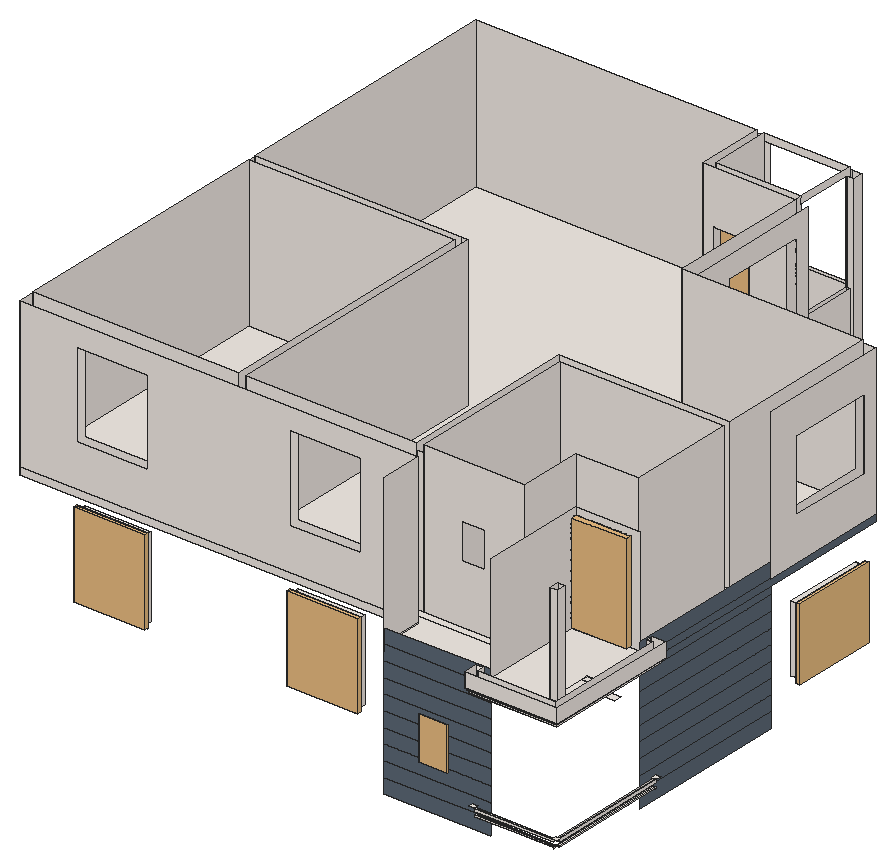
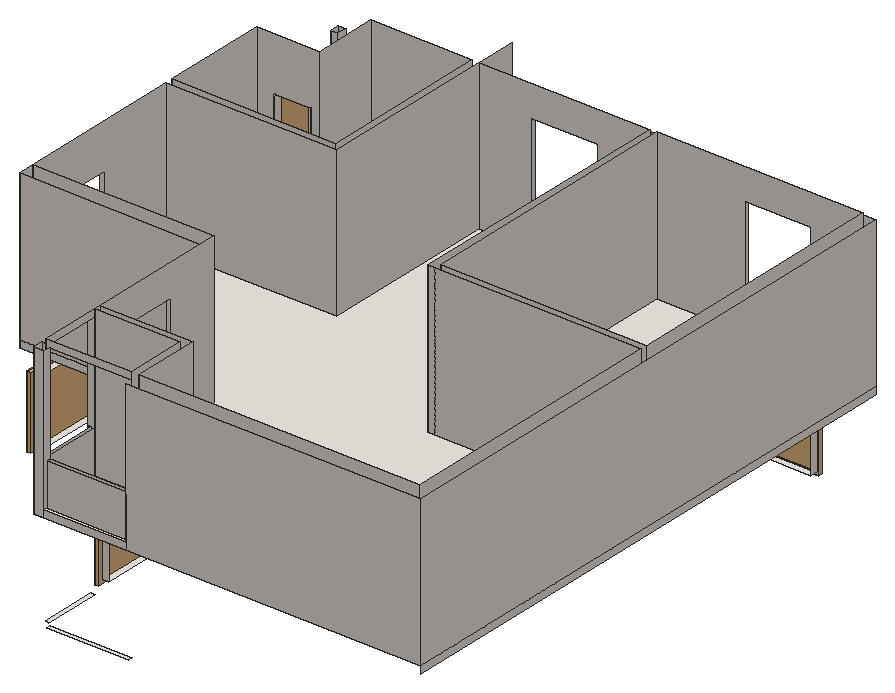
# SketchUp Ruby script. Lengths in inches.
U = 1.inch
M = Sketchup.active_model
def pt(a) = Geom::Point3d.new(a.map { |v| v * U })
def face(e, loops, mat)
  f = e.add_face(loops[0].map { |a| pt(a) })
  loops[1..].each { |l| e.add_face(l.map { |a| pt(a) }).erase! }
  f.material = f.back_material = mat if mat
  f
end
# faces: each face lists its corners as indices into pts; further lists are holes
def faces(e, pts, list, mat = nil) = list.each { |f| face(e, (f[0].is_a?(Array) ? f : [f]).map { |l| l.map { |i| pts[i] } }, mat) }
# xy, xz, yz: faces in a plane at the given z, y or x. An outline is a flat list of corners, or four numbers for a rectangle; further outlines are holes
def ring(l) = l.size == 4 ? [[l[0], l[1]], [l[2], l[1]], [l[2], l[3]], [l[0], l[3]]] : l.each_slice(2).to_a
def flat(e, list, mat, &to3) = list.each { |f| face(e, (f[0].is_a?(Array) ? f : [f]).map { |l| ring(l).map { |u, v| to3.(u, v) } }, mat) }
def xy(e, z, list, mat = nil) = flat(e, list, mat) { |x, y| [x, y, z] }
def xz(e, y, list, mat = nil) = flat(e, list, mat) { |x, z| [x, y, z] }
def yz(e, x, list, mat = nil) = flat(e, list, mat) { |y, z| [x, y, z] }
def lines(e, pts, list) = list.each { |a, b| e.add_line(pt(pts[a]), pt(pts[b])) }
# prism: a flat outline (further loops are holes) pulled along v
def prism(e, loops, v, mat = nil)
  f = face(e, loops, mat); d = Geom::Vector3d.new(v.map { |x| x * U })
  f.pushpull(f.normal.samedirection?(d) ? d.length : -d.length)
end
def box(e, o, s, mat = nil) = prism(e, [[o, [o[0] + s[0], o[1], o[2]], [o[0] + s[0], o[1] + s[1], o[2]], [o[0], o[1] + s[1], o[2]]]], [0, 0, s[2]], mat)
def at(x, y, z, deg = 0) = Geom::Transformation.translation(pt([x, y, z])) * Geom::Transformation.rotation(ORIGIN, Z_AXIS, deg.degrees)
def axes(o, x, y, z) = Geom::Transformation.new([*x, 0, *y, 0, *z, 0, *pt(o).to_a, 1])
def part(name) = M.definitions.add(name)
# library, detail: a bought-in or finely detailed component or shape, given as its bounding box
def library(name, o, s) = part(name).tap { |d| box(d.entities, o, s) }
def detail(e, o, s) = box(e.add_group.entities, o, s)
def put(e, d, t, mat = nil) = e.add_instance(d, t).tap { |i| i.material = mat if mat }
def group(e, t, mat = nil) = e.add_group.tap { |g| g.transformation = t; g.material = mat if mat }.entities
root = M.entities
M.materials.add("D01_Frost_White").color = [242, 235, 229]
M.materials.add("Denim_03_1K").color = [93, 106, 119]
c1 = library("mesh-163",[-551.08,-704.17,-20.03],[1929.24,1401.85,86.96])
c2 = part("Group11")
put(c2.entities,c1,at(0,0,0))
c3 = library("porta+4",[0.2,-5.42,1.33],[46.55,4.72,83.21])
xy(root,148.95,[[[432,9.26,498.04,11.26],[432.74,9.55,433.14,11.05],[434.88,9.55,435.28,11.05],[437.03,9.55,437.43,11.05],[439.17,9.55,439.57,11.05],[441.32,9.55,441.72,11.05],[443.46,9.55,443.86,11.05],[445.61,9.55,446.01,11.05],[447.76,9.55,448.16,11.05],[449.9,9.55,450.3,11.05],[452.05,9.55,452.45,11.05],[454.19,9.55,454.59,11.05],[456.34,9.55,456.74,11.05],[458.48,9.55,458.88,11.05],[460.63,9.55,461.03,11.05],[462.77,9.55,463.17,11.05],[464.92,9.55,465.32,11.05],[467.06,9.55,467.46,11.05],[469.21,9.55,469.61,11.05],[471.36,9.55,471.76,11.05],[473.5,9.55,473.9,11.05],[475.65,9.55,476.05,11.05],[477.79,9.55,478.19,11.05],[479.9375,9.55,480.34,11.05],[482.08,9.55,482.48,11.05],[484.23,9.55,484.63,11.05],[486.375,9.55,486.77,11.05],[488.52,9.55,488.92,11.05],[490.67,9.55,491.07,11.05],[492.8125,9.55,493.21,11.05],[494.96,9.55,495.36,11.05],[497.1,9.55,497.5,11.05]],[[498.875,12.05,500.875,113.6],[499.1,12.64,500.6,13.04],[499.1,15.15,500.6,15.55],[499.1,17.65,500.6,18.05],[499.1,20.16,500.6,20.56],[499.1,22.66,500.6,23.06],[499.1,25.16,500.6,25.5625],[499.1,27.67,500.6,28.07],[499.1,30.17,500.6,30.57],[499.1,32.67,500.6,33.07],[499.1,35.18,500.6,35.58],[499.1,37.68,500.6,38.08],[499.1,40.1875,500.6,40.59],[499.1,42.69,500.6,43.09],[499.1,45.19,500.6,45.59],[499.1,47.7,500.6,48.1],[499.1,50.2,500.6,50.6],[499.1,52.71,500.6,53.11],[499.1,55.21,500.6,55.61],[499.1,57.71,500.6,58.11],[499.1,60.22,500.6,60.62],[499.1,62.72,500.6,63.12],[499.1,65.22,500.6,65.625],[499.1,67.73,500.6,68.13],[499.1,70.23,500.6,70.63],[499.1,72.74,500.6,73.14],[499.1,75.24,500.6,75.64],[499.1,77.74,500.6,78.14],[499.1,80.25,500.6,80.65],[499.1,82.75,500.6,83.15],[499.1,85.25,500.6,85.65],[499.1,87.76,500.6,88.16],[499.1,90.26,500.6,90.66],[499.1,92.77,500.6,93.17],[499.1,95.27,500.6,95.67],[499.1,97.77,500.6,98.17],[499.1,100.28,500.6,100.68],[499.1,102.78,500.6,103.18],[499.1,105.28,500.6,105.68],[499.1,107.79,500.6,108.1875],[499.1,110.29,500.6,110.69],[499.1,112.8,500.6,113.2]]],"D01_Frost_White")
xy(root,149.95,[[432,9.26,498.04,11.26],[498.875,12.05,500.875,113.6]],"D01_Frost_White")
xy(root,152.81,[[432,9.26,498.04,11.26],[498.875,12.05,500.875,113.6]],"D01_Frost_White")
xy(root,154.81,[[432,9.26,498.04,11.26],[498.875,12.05,500.875,113.6]],"D01_Frost_White")
xy(root,156,[[428,8,432,12],[498.04,8.05,502.04,12.05],[498.04,113.6,502.04,117.6]],"D01_Frost_White")
xy(root,158,[[486,275,492,343]],"D01_Frost_White")
xy(root,162,[[333,477,336,525],[261,528,330,531]],"D01_Frost_White")
xy(root,164,[[62,54,108,60],[108,54,118,60],[242,54,288,60],[288,54,298,60]],"D01_Frost_White")
xy(root,165,[[333,396,339,462]],"D01_Frost_White")
xy(root,170,[[380,18,400,60]],"Denim_03_1K")
xy(root,202,[[380,18,400,60]],"Denim_03_1K")
xy(root,207,[[441,108,471,114],[264,471,294,477]],"D01_Frost_White")
xy(root,214,[[486,275,492,343]],"D01_Frost_White")
xy(root,231,[[333,396,339,462]],"D01_Frost_White")
xy(root,232,[[62,54,118,60],[242,54,298,60]],"D01_Frost_White")
xy(root,240,[[[448,16,494,98],[486,54,486.67,60,486,60]],[486,21.03,492,29],[486,29,486.67,54],[486.67,29,492,54],[486,54,486.67,60]],"D01_Frost_White")
xy(root,242,[[[428,8,428,16,440,16,440,106,494,106,494,118,502,118,502,8],[430,10,500,10,500,116,496,116,496,104,442,104,442,14,430,14]],[[430,10,430,14,442,14,442,104,496,104,496,116,500,116,500,10],[448,16,494,98]]],"D01_Frost_White")
xy(root,244,[[[427,7,427,17,439,17,439,107,493,107,493,119,503,119,503,7],[428,8,502,8,502,118,494,118,494,106,440,106,440,16,428,16]]],"D01_Frost_White")
xy(root,246,[[[426,6,426,18,438,18,438,108,492,108,492,120,504,120,504,6],[427,7,503,7,503,119,493,119,493,107,439,107,439,17,427,17]],[348,18,348,54,18,54,18,528,255,528,255,471,333,471,333,351,486,351,486,114,432,114,432,60,438,60,438,18],[12,54,18,528],[486,54,486,60,486.67,60],[486,54,486.67,60,486.67,54],
  [486.67,54,492,60],[486,108,492,351],[333,351,492,351,492,357,339,357,339,477,261,477,261,528,255,528,255,471,333,471],[261,477,333,528],[333,477,339,525],
  [333,525,339,534],[12,528,261,534],[261,528,330,534],[330,528,333,534]],"D01_Frost_White")
xy(root,247.18,[[18,60,18,528,255,528,255,471,333,471,333,351,486,351,486,60]],"D01_Frost_White")
xy(root,252,[[[432,12,498,12,498,114,492,114,492,108,438,108,438,18,432,18],[486,21.03,492,60]],[486,21.03,492,54],[486,29,492,60],[18,60,192,288],[198,60,342,60,342,210,486,210,486,351,333,351,333,471,255,471,255,528,18,528,18,294,198,294],
  [348,60,433.5,60,433.5,114,486,114,486,204,348,204],[261,477,333,528],[336,477,339,525],[261,531,330,534]],"D01_Frost_White")
xy(root,255,[[441,108,471,114],[441,114,471,115.5],[264,471,294,477]],"D01_Frost_White")
xz(root,6,[[426,246,504,258]],"D01_Frost_White")
xz(root,7,[[427,244,503,246]],"D01_Frost_White")
xz(root,8,[[428,242,502,244]],"D01_Frost_White")
xz(root,9.26,[[432,148.95,498.04,149.95],[432,152.81,498.04,154.81]],"D01_Frost_White")
xz(root,11.26,[[432,148.95,498.04,149.95],[432,152.81,498.04,154.81]],"D01_Frost_White")
xz(root,12,[[432,252,498,258]],"D01_Frost_White")
xz(root,16,[[448,240,494,242],[428,242,440,244]],"D01_Frost_White")
xz(root,17,[[427,244,439,246]],"D01_Frost_White")
xz(root,18,[[348,132.6,438,145.2],[348,145.2,438,157.8],[348,157.8,438,157.8,438,170.4,402,170.4,402,168,378,168,378,170.4,348,170.4],[[378,168,402,204],[380,170,400,202]],[348,170.4,378,183],
  [402,170.4,438,183],[348,183,378,195.6],[402,183,438,195.6],[348,195.6,378,195.6,378,204,402,204,402,195.6,438,195.6,438,208.2,348,208.2],[348,208.2,438,220.8],
  [348,220.8,438,233.4],[348,233.4,438,246],[348,246,426,246,426,258,432,258,432,252,438,252,438,258.6,348,258.6]],"Denim_03_1K")
xz(root,21.03,[[486,252,492,336]],"D01_Frost_White")
xz(root,29,[[486,252,492,336]],"D01_Frost_White")
xz(root,54,[[[60,162,120,234],[62,164,118,232]],[[240,162,300,234],[242,164,298,232]],[12,240,348,246],[486,240,486.67,246],[486.67,240,492,246],
  [[12,246,348,372],[60,282,120,354],[240,282,300,354]],[486,246,492,252]],"D01_Frost_White")
xz(root,60,[[486,240,486.67,246],[486,246,492,252],[[18,252,192,378],[62,284,118,352]],[[198,252,342,378],[242,284,298,352]],[342,252,348,372],
  [[348,252,433.5,378],[380,302,400,332.2]]],"D01_Frost_White")
xz(root,98,[[448,240,486,242],[486,240,494,242]],"D01_Frost_White")
xz(root,106,[[440,242,486,244],[486,242,494,244]],"D01_Frost_White")
xz(root,107,[[439,244,486,246],[486,244,493,246]],"D01_Frost_White")
xz(root,108,[[474,252,492,252,492,342,438,342,438,336,474,336],[[438,252,474,336],[441,255,471,333]]],"D01_Frost_White")
xz(root,113.6,[[498.875,147.95,500.875,148.95]],"D01_Frost_White")
xz(root,114,[[[433.5,252,486,378],[441,255,471,333]],[492,252,498,258]],"D01_Frost_White")
xz(root,118,[[494,242,502,244]],"D01_Frost_White")
xz(root,119,[[493,244,503,246]],"D01_Frost_White")
xz(root,120,[[492,246,504,258]],"D01_Frost_White")
xz(root,204,[[348,252,486,378]],"D01_Frost_White")
xz(root,210,[[342,252,486,378]],"D01_Frost_White")
xz(root,275,[[486,158,492,214]],"D01_Frost_White")
xz(root,288,[[18,252,192,378]],"D01_Frost_White")
xz(root,294,[[18,252,192,378],[192,252,198,378]],"D01_Frost_White")
xz(root,343,[[486,158,492,214]],"D01_Frost_White")
xz(root,351,[[333,246,486,247.18],[333,252,486,378]],"D01_Frost_White")
xz(root,357,[[339,240,492,246],[339,246,492,372]],"D01_Frost_White")
xz(root,396,[[333,165,339,231]],"D01_Frost_White")
xz(root,462,[[333,165,339,231]],"D01_Frost_White")
xz(root,471,[[255,246,333,247.18],[[255,252,333,378],[264,255,294,333]]],"D01_Frost_White")
xz(root,477,[[297,252,297,336,261,336,261,378,333,378,333,252],[[261,252,297,336],[264,255,294,333]],[336,252,339,288]],"D01_Frost_White")
xz(root,525,[[336,252,339,252,339,372,333,372,333,288,336,288]],"D01_Frost_White")
xz(root,528,[[18,246,255,247.18],[18,252,255,378],[261,252,330,288],[330,252,333,252,333,378,261,378,261,372,330,372]],"D01_Frost_White")
xz(root,531,[[261,252,330,288]],"D01_Frost_White")
xz(root,534,[[12,246,261,372],[261,246,330,252],[330,246,339,372]],"D01_Frost_White")
yz(root,12,[[54,240,534,246],[54,246,534,372]],"D01_Frost_White")
yz(root,18,[[60,246,528,247.18],[60,252,288,378],[294,252,528,378]],"D01_Frost_White")
yz(root,62,[[54,164,60,222],[54,222,60,232]],"D01_Frost_White")
yz(root,118,[[54,164,60,232]],"D01_Frost_White")
yz(root,192,[[60,252,288,378]],"D01_Frost_White")
yz(root,198,[[60,252,294,378]],"D01_Frost_White")
yz(root,242,[[54,164,60,222],[54,222,60,232]],"D01_Frost_White")
yz(root,255,[[471,246,528,247.18],[471,252,528,378]],"D01_Frost_White")
yz(root,261,[[477,252,528,378],[531,252,534,288]],"D01_Frost_White")
yz(root,264,[[471,255,477,333]],"D01_Frost_White")
yz(root,294,[[471,255,477,333]],"D01_Frost_White")
yz(root,298,[[54,164,60,232]],"D01_Frost_White")
yz(root,330,[[531,252,531,288,528,288,528,372,534,372,534,252]],"D01_Frost_White")
yz(root,333,[[351,246,471,247.18],[[351,252,471,378],[396,285,462,351]],[471,252,477,378],[477,252,525,288],[525,252,525,372,477,372,477,378,528,378,528,252]],"D01_Frost_White")
yz(root,336,[[477,252,525,288]],"D01_Frost_White")
yz(root,339,[[[393,162,465,234],[396,165,462,231]],[357,240,477,246],[[357,246,477,372],[393,282,465,354]],[477,246,525,252],[525,246,534,372]],"D01_Frost_White")
yz(root,342,[[60,252,210,378]],"D01_Frost_White")
yz(root,348,[[18,240,54,246],[18,246,54,372],[60,252,204,378]],"D01_Frost_White")
yz(root,380,[[18,170,60,170.4],[18,170.4,60,183],[18,183,60,195.6],[18,195.6,60,202]],"Denim_03_1K")
yz(root,400,[[18,170,60,170.4],[18,170.4,60,183],[18,183,60,195.6],[18,195.6,60,202]],"Denim_03_1K")
yz(root,426,[[6,246,18,258]],"D01_Frost_White")
yz(root,427,[[7,244,17,246]],"D01_Frost_White")
yz(root,428,[[8,242,16,244]],"D01_Frost_White")
yz(root,432,[[12,252,18,258]],"D01_Frost_White")
yz(root,433.5,[[60,252,114,378]],"D01_Frost_White")
yz(root,438,[[18,252,108,342]],"D01_Frost_White")
yz(root,439,[[17,244,60,246],[60,244,107,246]],"D01_Frost_White")
yz(root,440,[[16,242,60,244],[60,242,106,244]],"D01_Frost_White")
yz(root,441,[[108,255,114,333],[114,255,115.5,333]],"D01_Frost_White")
yz(root,448,[[16,240,60,242],[60,240,98,242]],"D01_Frost_White")
yz(root,471,[[108,255,114,333],[114,255,115.5,333]],"D01_Frost_White")
yz(root,486,[[54,240,60,246],[54,246,60,252],[108,246,351,247.18],[21.03,252,29,336],[114,252,204,378],
  [[210,252,351,378],[275,284,343,340]]],"D01_Frost_White")
yz(root,486.67,[[54,240,60,246]],"D01_Frost_White")
yz(root,492,[[[273,156,345,216],[275,158,343,214]],[54,246,60,252],[[246,246,357,372],[273,282,345,342]],[21.03,252,29,336]],"D01_Frost_White")
yz(root,492,[[108,132.6,246,145.2],[108,145.2,246,157.8],[108,157.8,246,170.4],[108,170.4,246,183],[108,183,246,195.6],
  [108,195.6,246,208.2],[108,208.2,246,220.8],[108,220.8,246,233.4],[108,233.4,246,240],[108,240,357,246],
  [120,246,246,246,246,258.6,108,258.6,108,252,114,252,114,258,120,258]],"Denim_03_1K")
yz(root,493,[[107,244,119,246]],"D01_Frost_White")
yz(root,494,[[16,240,98,242],[106,242,118,244]],"D01_Frost_White")
yz(root,498,[[12,252,114,258]],"D01_Frost_White")
yz(root,498.04,[[9.26,147.95,11.26,148.95]],"D01_Frost_White")
yz(root,498.875,[[12.05,148.95,113.6,149.95],[12.05,152.81,113.6,154.81]],"D01_Frost_White")
yz(root,500.875,[[12.05,148.95,113.6,149.95],[12.05,152.81,113.6,154.81]],"D01_Frost_White")
yz(root,502,[[8,242,118,244]],"D01_Frost_White")
yz(root,503,[[7,244,119,246]],"D01_Frost_White")
yz(root,504,[[6,246,120,258]],"D01_Frost_White")
p = [[486,54,246],[486.67,60,246],[486.67,60,240],[486,54,240]]
faces(root,p,[[0,1,2,3]],"D01_Frost_White")
put(root,c2,axes([494.63,324.55,185.79],[0,-0.0374,0],[0,0,0.04331],[-0.03937,0,0]))
put(root,c2,axes([341.63,444.55,197.74],[0,-0.0374,0],[0,0,0.05197],[-0.03937,0,0]))
put(root,c2,axes([77.14,53.21,198.29],[0.0311,0,0],[0,0,0.05118],[0,-0.03937,0]))
put(root,c2,axes([257.14,53.21,198.29],[0.0311,0,0],[0,0,0.05118],[0,-0.03937,0]))
put(root,c2,axes([384.83,17.76,186.04],[0.0124,0,0],[0,0,0.02575],[0,-0.01181,0]))
put(root,c3,at(437.8,108.7,251.46))
put(root,c3,at(250.25,482.42,251.46))
